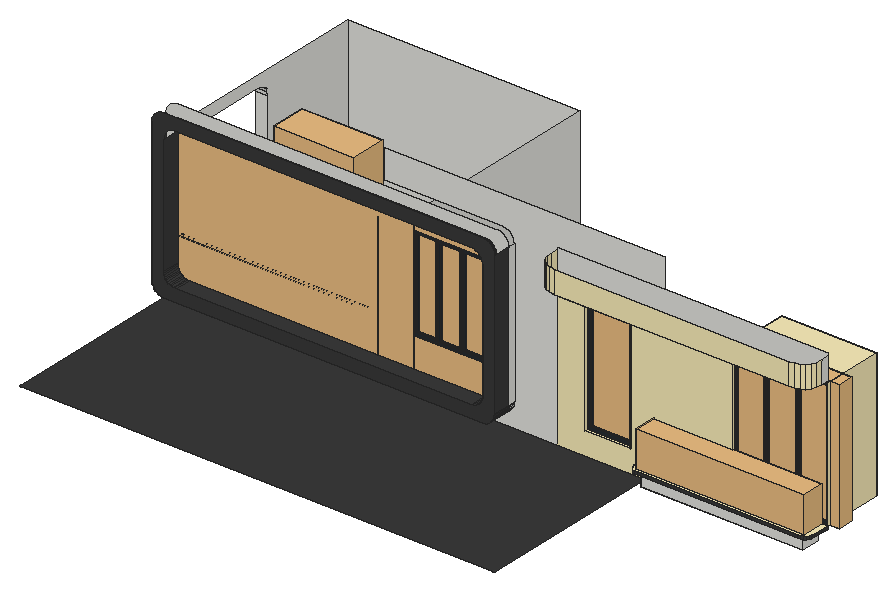
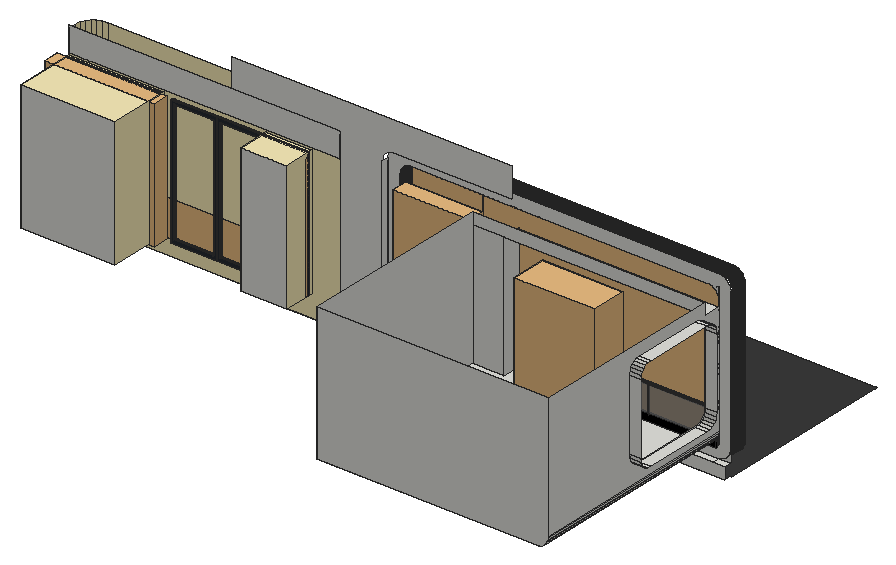
# SketchUp Ruby script. Lengths in inches.
U = 1.inch
M = Sketchup.active_model
def pt(a) = Geom::Point3d.new(a.map { |v| v * U })
def face(e, loops, mat)
  f = e.add_face(loops[0].map { |a| pt(a) })
  loops[1..].each { |l| e.add_face(l.map { |a| pt(a) }).erase! }
  f.material = f.back_material = mat if mat
  f
end
# faces: each face lists its corners as indices into pts; further lists are holes
def faces(e, pts, list, mat = nil) = list.each { |f| face(e, (f[0].is_a?(Array) ? f : [f]).map { |l| l.map { |i| pts[i] } }, mat) }
# xy, xz, yz: faces in a plane at the given z, y or x. An outline is a flat list of corners, or four numbers for a rectangle; further outlines are holes
def ring(l) = l.size == 4 ? [[l[0], l[1]], [l[2], l[1]], [l[2], l[3]], [l[0], l[3]]] : l.each_slice(2).to_a
def flat(e, list, mat, &to3) = list.each { |f| face(e, (f[0].is_a?(Array) ? f : [f]).map { |l| ring(l).map { |u, v| to3.(u, v) } }, mat) }
def xy(e, z, list, mat = nil) = flat(e, list, mat) { |x, y| [x, y, z] }
def xz(e, y, list, mat = nil) = flat(e, list, mat) { |x, z| [x, y, z] }
def yz(e, x, list, mat = nil) = flat(e, list, mat) { |y, z| [x, y, z] }
def lines(e, pts, list) = list.each { |a, b| e.add_line(pt(pts[a]), pt(pts[b])) }
# prism: a flat outline (further loops are holes) pulled along v
def prism(e, loops, v, mat = nil)
  f = face(e, loops, mat); d = Geom::Vector3d.new(v.map { |x| x * U })
  f.pushpull(f.normal.samedirection?(d) ? d.length : -d.length)
end
def box(e, o, s, mat = nil) = prism(e, [[o, [o[0] + s[0], o[1], o[2]], [o[0] + s[0], o[1] + s[1], o[2]], [o[0], o[1] + s[1], o[2]]]], [0, 0, s[2]], mat)
def at(x, y, z, deg = 0) = Geom::Transformation.translation(pt([x, y, z])) * Geom::Transformation.rotation(ORIGIN, Z_AXIS, deg.degrees)
def axes(o, x, y, z) = Geom::Transformation.new([*x, 0, *y, 0, *z, 0, *pt(o).to_a, 1])
def part(name) = M.definitions.add(name)
# library, detail: a bought-in or finely detailed component or shape, given as its bounding box
def library(name, o, s) = part(name).tap { |d| box(d.entities, o, s) }
def detail(e, o, s) = box(e.add_group.entities, o, s)
def put(e, d, t, mat = nil) = e.add_instance(d, t).tap { |i| i.material = mat if mat }
def group(e, t, mat = nil) = e.add_group.tap { |g| g.transformation = t; g.material = mat if mat }.entities
root = M.entities
M.materials.add("0899 AP 7833 SUNKISSED").color = [249, 236, 185]
M.materials.add("Glass Railing Color").color = [198, 198, 198]
M.materials.add("Railing Glass").color = [63, 150, 137]
M.materials["Railing Glass"].alpha = 0.13
M.materials.add("Wine2").color = [0, 0, 0]
M.materials["Wine2"].alpha = 0
M.materials.add("[0130_Gainsboro]").color = [39, 45, 50]
M.materials.add("[Color M07]").color = [58, 58, 58]
M.materials.add("[Color M09]").color = [0, 0, 0]
M.materials.add("[Translucent Glass Gray]").color = [128, 128, 128]
M.materials["[Translucent Glass Gray]"].alpha = 0.5
M.materials.add("[Wood Veneer 02]").color = [190, 128, 91]
c1 = part("Window sash")
xy(c1.entities,0,[[0,-0.98,43.07,0],[0,0,43.07,1.4]],"[0130_Gainsboro]")
xy(c1.entities,0.3,[[0.3,-1.43,42.77,-0.98]],"[0130_Gainsboro]")
xy(c1.entities,2.95,[[2.95,-1.43,40.12,-0.63],[2.95,-0.63,40.12,0],[2.95,0,40.12,0.64],[2.95,0.64,40.12,1.4]],"[0130_Gainsboro]")
xy(c1.entities,3.54,[[3.54,-0.63,39.53,0],[3.54,0,39.53,0.64]],"[0130_Gainsboro]")
xy(c1.entities,111.8125,[[3.54,-0.63,39.53,0],[3.54,0,39.53,0.64]],"[0130_Gainsboro]")
xy(c1.entities,112.4,[[2.95,-1.43,40.12,-0.63],[2.95,-0.63,40.12,0],[2.95,0,40.12,0.64],[2.95,0.64,40.12,1.4]],"[0130_Gainsboro]")
xy(c1.entities,115.05,[[0.3,-1.43,42.77,-0.98]],"[0130_Gainsboro]")
xy(c1.entities,115.35,[[0,-0.98,43.07,0],[0,0,43.07,1.4]],"[0130_Gainsboro]")
xz(c1.entities,-1.43,[[[0.3,0.3,42.77,115.05],[2.95,2.95,40.12,112.4]]],"[0130_Gainsboro]")
xz(c1.entities,-0.98,[[[0,0,43.07,115.35],[0.3,0.3,42.77,115.05]]],"[0130_Gainsboro]")
xz(c1.entities,-0.63,[[[2.95,2.95,40.12,112.4],[3.54,3.54,39.53,111.8125]]],"[0130_Gainsboro]")
xz(c1.entities,0,[[3.54,3.54,39.53,111.8125]],"Wine2")
xz(c1.entities,0,[[[0,0,43.07,115.35],[2.95,2.95,40.12,112.4]],[[2.95,2.95,40.12,112.4],[3.54,3.54,39.53,111.8125]]],"[0130_Gainsboro]")
xz(c1.entities,0.64,[[[2.95,2.95,40.12,112.4],[3.54,3.54,39.53,111.8125]]],"[0130_Gainsboro]")
xz(c1.entities,1.4,[[[0,0,43.07,115.35],[2.95,2.95,40.12,112.4]]],"[0130_Gainsboro]")
yz(c1.entities,0,[[-0.98,0,0,115.35],[0,0,1.4,115.35]],"[0130_Gainsboro]")
yz(c1.entities,0.3,[[-1.43,0.3,-0.98,115.05]],"[0130_Gainsboro]")
yz(c1.entities,2.95,[[-1.43,2.95,-0.63,112.4],[-0.63,2.95,0,112.4],[0,2.95,0.64,112.4],[0.64,2.95,1.4,112.4]],"[0130_Gainsboro]")
yz(c1.entities,3.54,[[-0.63,3.54,0,111.8125],[0,3.54,0.64,111.8125]],"[0130_Gainsboro]")
yz(c1.entities,39.53,[[-0.63,3.54,0,111.8125],[0,3.54,0.64,111.8125]],"[0130_Gainsboro]")
yz(c1.entities,40.12,[[-1.43,2.95,-0.63,112.4],[-0.63,2.95,0,112.4],[0,2.95,0.64,112.4],[0.64,2.95,1.4,112.4]],"[0130_Gainsboro]")
yz(c1.entities,42.77,[[-1.43,0.3,-0.98,115.05]],"[0130_Gainsboro]")
yz(c1.entities,43.07,[[-0.98,0,0,115.35],[0,0,1.4,115.35]],"[0130_Gainsboro]")
c2 = part("Three-panel window")
put(c2.entities,c1,axes([90.57,1.43,0],[1.05148,0,0],[0,1,0],[0,0,1]))
put(c2.entities,c1,axes([0,1.43,0],[1.05148,0,0],[0,1,0],[0,0,1]))
put(c2.entities,c1,axes([45.29,1.43,0],[1.05148,0,0],[0,1,0],[0,0,1]))
c3 = library("шторы раздвинутые\#1",[23.6875,-79.37,-3.6],[68.3125,79.85,10.87])
c4 = library("Glass Railing",[-110.8125,-14.6875,0],[111.5625,15.1875,24])
c5 = part("Group\#61")
p = [[0,1.89,0.38],[0,1.89,1.61],[0,0.72,0],[0,0,0.99],[0,0.72,1.99]]
lines(c5.entities,p,[[0,1],[2,0],[3,2],[4,3],[1,4]])
c6 = part("Pleated curtain panel")
p = [[20.45,2.26,80],[20.78,2.41,80]]
lines(c6.entities,p,[[0,1]])
detail(c6.entities,[0,1.93,2.7],[20.05,3.87,77.3])
put(c6.entities,c5,at(9.77,5.02,80,-180))
put(c6.entities,c5,at(11.91,5.02,80,-180))
put(c6.entities,c5,at(13.54,5.02,80,-180))
put(c6.entities,c5,at(7.29,5.02,80,-180))
put(c6.entities,c5,at(6.18,5.02,80,-180))
put(c6.entities,c5,at(8.69,5.02,80,-180))
put(c6.entities,c5,at(17.42,5.04,80,-180))
put(c6.entities,c5,at(18.86,5.04,80,-180))
put(c6.entities,c5,at(15.09,5.02,80,-180))
put(c6.entities,c5,at(16.66,5.04,80,-180))
put(c6.entities,c5,at(2.54,5.02,80,-180))
put(c6.entities,c5,at(1.38,5.02,80,-180))
put(c6.entities,c5,at(4.1,5.02,80,-180))
c7 = part("Glass Rail Spacer")
box(c7.entities,[-0.5,-0.25,0],[1,0.5,1],"Glass Railing Color")
c8 = part("Group19\#1")
prism(c8.entities,[[[0.54,0,1.27],[0.38,0,1.39],[0.21,0,1.47],[0.01,0,1.5],[-0.18,0,1.48],[-0.37,0,1.41],[-0.52,0,1.29],[-0.64,0,1.13],[-0.72,0,0.96],[-0.75,0,0.76],[-0.73,0,0.57],[-0.66,0,0.38],[-0.54,0,0.23],[-0.38,0,0.11],[-0.21,0,0.03],[-0.01,0,0],[0.18,0,0.02],[0.37,0,0.09],[0.52,0,0.21],[0.64,0,0.37],[0.72,0,0.54],[0.75,0,0.74],[0.73,0,0.93],[0.66,0,1.12]]],[0,136.79,0],"[Color M09]")
c9 = part("Group22\#2")
prism(c9.entities,[[[0.25,0,5],[0.25,0,4],[-0.25,0,4],[-0.25,0,5],[-0.5,0,5],[-0.5,0,0],[0.5,0,0],[0.5,0,5]]],[0,136.79,0],"[Color M09]")
c10 = part("Group23\#2")
box(c10.entities,[-0.1875,0,0],[0.375,44.26,18.5],"[Translucent Glass Gray]")
c11 = part("Group24\#2")
box(c11.entities,[-0.1875,0,0],[0.375,44.26,18.5],"[Translucent Glass Gray]")
c12 = part("Group25\#2")
box(c12.entities,[-0.1875,0,0],[0.375,44.26,18.5],"[Translucent Glass Gray]")
c13 = part("Glass Railing\#2")
put(c13.entities,c7,at(0,0,4,180))
put(c13.entities,c7,at(-45.26,0,4,180))
put(c13.entities,c7,at(-90.53,0,4,180))
put(c13.entities,c7,at(-135.79,0,4,180))
put(c13.entities,c8,at(0.5,0,22.5,90),"[Color M09]")
put(c13.entities,c9,at(0.5,0,0,90),"Glass Railing Color")
put(c13.entities,c10,at(-0.5,0,4,90),"[Translucent Glass Gray]")
put(c13.entities,c11,at(-45.76,0,4,90),"Railing Glass")
put(c13.entities,c12,at(-91.03,0,4,90),"Railing Glass")
c14 = library("Group24\#3",[-80,-48,0],[160,96,0.25])
c15 = library("Group160\#2",[-28,-10,0],[56,20,0.25])
c16 = library("sWING-1250",[0,0,16],[54.55,24,105.18])
c17 = part("Group253\#1")
prism(c17.entities,[[[-3,37.93,0],[-3,-38,0],[-4,-38,0],[-4,26,0],[-4,38,0]]],[0,0,0.25])
c18 = part("Group254\#1")
xy(c18.entities,0,[[-2.8125,-38,-2.8125,37.9,-1.93,37.73,-1.8125,37.6875,-1.8125,-38]])
xy(c18.entities,0.25,[[-2.8125,-38,-1.8125,-38,-1.8125,37.6875,-1.93,37.73,-2.8125,37.9]])
xz(c18.entities,-38,[[-2.8125,0,-1.8125,0.25]])
yz(c18.entities,-2.8125,[[-38,0,37.9,0.25]])
yz(c18.entities,-1.8125,[[-38,0,37.6875,0.25]])
c19 = part("Group255\#1")
xy(c19.entities,0,[[-1.625,-38,-1.625,37.625,-0.9375,37.39,-0.625,37.24,-0.625,-38]])
xy(c19.entities,0.25,[[-1.625,-38,-0.625,-38,-0.625,37.24,-0.9375,37.39,-1.625,37.625]])
xz(c19.entities,-38,[[-1.625,0,-0.625,0.25]])
yz(c19.entities,-1.625,[[-38,0,37.625,0.25]])
yz(c19.entities,-0.625,[[-38,0,37.24,0.25]])
c20 = part("Group256\#1")
xy(c20.entities,0,[[-0.4375,-38,-0.4375,37.14,0,36.93,0.5625,36.55,0.5625,-38]])
xy(c20.entities,0.25,[[-0.4375,-38,0.5625,-38,0.5625,36.55,0,36.93,-0.4375,37.14]])
xz(c20.entities,-38,[[-0.4375,0,0.5625,0.25]])
yz(c20.entities,-0.4375,[[-38,0,37.14,0.25]])
yz(c20.entities,0.5625,[[-38,0,36.55,0.25]])
c21 = part("Group257\#1")
xy(c21.entities,0,[[0.75,-38,0.75,36.43,0.87,36.35,1.66,35.66,1.75,35.55,1.75,-38]])
xy(c21.entities,0.25,[[0.75,-38,1.75,-38,1.75,35.55,1.66,35.66,0.87,36.35,0.75,36.43]])
xz(c21.entities,-38,[[0.75,0,1.75,0.25]])
yz(c21.entities,0.75,[[-38,0,36.43,0.25]])
yz(c21.entities,1.75,[[-38,0,35.55,0.25]])
c22 = part("Group258\#1")
xy(c22.entities,0,[[1.9375,-38,1.9375,35.34,2.35,34.87,2.93,34,2.9375,33.98,2.9375,-38]])
xy(c22.entities,0.25,[[1.9375,-38,2.9375,-38,2.9375,33.98,2.93,34,2.35,34.87,1.9375,35.34]])
yz(c22.entities,1.9375,[[-38,0,35.34,0.25]])
yz(c22.entities,2.9375,[[-38,0,33.98,0.25]])
c23 = part("Group259\#1")
xy(c23.entities,0,[[3.125,-38,3.125,33.6,3.39,33.0625,3.73,32.07,3.93,31.04,4,30,4,-38]])
xy(c23.entities,0.25,[[3.125,-38,4,-38,4,30,3.93,31.04,3.73,32.07,3.39,33.0625,3.125,33.6]])
yz(c23.entities,3.125,[[-38,0,33.6,0.25]])
c24 = part("Group251\#2")
put(c24.entities,c17,at(0,0,0))
put(c24.entities,c18,at(0,0,0))
put(c24.entities,c19,at(0,0,0))
put(c24.entities,c20,at(0,0,0))
put(c24.entities,c21,at(0,0,0))
put(c24.entities,c22,at(0,0,0))
put(c24.entities,c23,at(0,0,0))
c25 = library("Group209\#2",[-24,-6,0],[48,12,0.25])
xy(root,135,[[2.06,0,319.94,0,320.57,0.06,321.09,0.23,321.49,0.51,321.77,0.91,321.94,1.43,322,2.06,322,123.1875,321,123.1875,321,128.1875,1,128.1875,1,123.1875,0,123.1875,0,2.06,0.06,1.43,0.23,0.91,0.51,0.51,0.91,0.23,1.43,0.06],[321,123.1875,322,128.1875]],"[Color M07]")
xy(root,139,[[329.02,115.4375,438.6,128.1875]])
xy(root,143,[[1,123.1875,9,128.1875],[9,123.1875,225,128.1875]])
xy(root,143,[[9,111.1875,225,123.1875]],"[Color M07]")
xy(root,148,[[330.04,111.1875,328.1,111.36,326.51,111.89,325.28,112.78,324.39,114.01,323.92,115.4375,323.86,115.6,323.6875,117.54,323.6875,128.1875,329.02,128.1875,329.02,115.4375,444.77,115.4375,444.29,114.01,443.41,112.78,442.18,111.89,440.59,111.36,438.65,111.1875]])
xy(root,150,[[330.04,111.1875,438.65,111.1875,440.59,111.36,442.18,111.89,443.41,112.78,444.29,114.01,444.77,115.4375,444.82,115.6,445,117.54,445,128.1875,438.6,128.1875,438.6,115.4375,329.02,115.4375,329.02,128.1875,323.6875,128.1875,323.6875,117.54,323.86,115.6,323.92,115.4375,324.39,114.01,325.28,112.78,326.51,111.89,328.1,111.36],[280.5,128.1875,311.5,149.5],[380.875,128.1875,445,169.5625]],"0899 AP 7833 SUNKISSED")
xy(root,151,[[17,123.1875,144.79,123.1875,144.79,135.1875,166.1,135.1875,166.1,267.1875,17,267.1875]])
xy(root,151,[[17,111.1875,217,123.1875]],"[Color M07]")
xy(root,171,[[169,123.1875,217,132.9375],[1,143.3,9,191.01]])
xy(root,235,[[9,123.1875,144.79,135.1875],[169,123.1875,217,132.9375],[1,143.3,9,191.01]])
xy(root,236.98,[[280.5,128.1875,311.5,149.5],[380.875,128.1875,445,169.5625]],"0899 AP 7833 SUNKISSED")
xy(root,238,[[274.28,111.1875,270.45,111.52,267.32,112.52,264.88,114.1875,263.14,116.52,262.1,119.52,261.75,123.1875,261.75,128.1875,445,128.1875,445,123.1875,444.65,119.52,443.61,116.52,441.87,114.1875,439.43,112.52,436.3,111.52,432.47,111.1875]],"0899 AP 7833 SUNKISSED")
xz(root,111.1875,[[274.28,238,432.47,253.0625]],"0899 AP 7833 SUNKISSED")
xz(root,111.1875,[[[9,143,225,143,226.04,143.07,227.07,143.27,228.0625,143.61,229,144.07,229.87,144.65,230.66,145.34,231.35,146.13,231.93,147,232.39,147.9375,232.73,148.93,232.93,149.96,233,151,233,247,232.93,248.04,232.73,249.07,232.39,250.0625,231.93,251,231.35,251.87,230.66,252.66,229.87,253.35,229,253.93,228.0625,254.39,227.07,254.73,226.04,254.93,225,255,9,255,7.96,254.93,6.93,254.73,5.9375,254.39,5,253.93,4.13,253.35,3.34,252.66,2.65,251.87,2.07,251,1.61,250.0625,1.27,249.07,1.07,248.04,1,247,1,151,1.07,149.96,1.27,148.93,1.61,147.9375,2.07,147,2.65,146.13,3.34,145.34,4.13,144.65,5,144.07,5.9375,143.61,6.93,143.27,7.96,143.07],[17,151,15.96,151.07,14.93,151.27,13.9375,151.61,13,152.07,12.13,152.65,11.34,153.34,10.65,154.13,10.07,155,9.61,155.9375,9.27,156.93,9.07,157.96,9,159,9,239,9.07,240.04,9.27,241.07,9.61,242.0625,10.07,243,10.65,243.87,11.34,244.66,12.13,245.35,13,245.93,13.9375,246.39,14.93,246.73,15.96,246.93,17,247,217,247,218.04,246.93,219.07,246.73,220.0625,246.39,221,245.93,221.87,245.35,222.66,244.66,223.35,243.87,223.93,243,224.39,242.0625,224.73,241.07,224.93,240.04,225,239,225,159,224.93,157.96,224.73,156.93,224.39,155.9375,223.93,155,223.35,154.13,222.66,153.34,221.87,152.65,221,152.07,220.0625,151.61,219.07,151.27,218.04,151.07,217,151]],[330.04,148,438.65,150]],"[Color M07]")
xz(root,115.4375,[[329.02,139,438.6,148],[329.02,148,438.6,150]])
xz(root,123.1875,[[1,143,9,143,7.96,143.07,6.93,143.27,5.9375,143.61,5,144.07,4.13,144.65,3.34,145.34,2.65,146.13,2.07,147,1.61,147.9375,1.27,148.93,1.07,149.96,1,151],[[9,143,7.96,143.07,6.93,143.27,5.9375,143.61,5,144.07,4.13,144.65,3.34,145.34,2.65,146.13,2.07,147,1.61,147.9375,1.27,148.93,1.07,149.96,1,151,1,247,1.07,248.04,1.27,249.07,1.61,250.0625,2.07,251,2.65,251.87,3.34,252.66,4.13,253.35,5,253.93,5.9375,254.39,6.93,254.73,7.96,254.93,9,255,225,255,226.04,254.93,227.07,254.73,228.0625,254.39,229,253.93,229.87,253.35,230.66,252.66,231.35,251.87,231.93,251,232.39,250.0625,232.73,249.07,232.93,248.04,233,247,233,151,232.93,149.96,232.73,148.93,232.39,147.9375,231.93,147,231.35,146.13,230.66,145.34,229.87,144.65,229,144.07,228.0625,143.61,227.07,143.27,226.04,143.07,225,143],[17,151,217,151,218.04,151.07,219.07,151.27,220.0625,151.61,221,152.07,221.87,152.65,222.66,153.34,223.35,154.13,223.93,155,224.39,155.9375,224.73,156.93,224.93,157.96,225,159,225,239,224.93,240.04,224.73,241.07,224.39,242.0625,223.93,243,223.35,243.87,222.66,244.66,221.87,245.35,221,245.93,220.0625,246.39,219.07,246.73,218.04,246.93,217,247,17,247,15.96,246.93,14.93,246.73,13.9375,246.39,13,245.93,12.13,245.35,11.34,244.66,10.65,243.87,10.07,243,9.61,242.0625,9.27,241.07,9.07,240.04,9,239,9,159,9.07,157.96,9.27,156.93,9.61,155.9375,10.07,155,10.65,154.13,11.34,153.34,12.13,152.65,13,152.07,13.9375,151.61,14.93,151.27,15.96,151.07]]])
xz(root,128.1875,[[1,135,261.75,135,261.75,255,334.71,255,334.71,274.625,145.5625,274.625,145.5625,255,225,255,226.04,254.93,227.07,254.73,228.0625,254.39,229,253.93,229.87,253.35,230.66,252.66,231.35,251.87,231.93,251,232.39,250.0625,232.73,249.07,232.93,248.04,233,247,233,151,232.93,149.96,232.73,148.93,232.39,147.9375,231.93,147,231.35,146.13,230.66,145.34,229.87,144.65,229,144.07,228.0625,143.61,227.07,143.27,226.04,143.07,225,143,1,143],[323.6875,148,329.02,150],[261.75,238,445,255]])
xz(root,128.1875,[[[261.75,135,323.6875,135,323.6875,150,329.02,150,329.02,139,438.6,139,438.6,150,380.875,150,380.875,236.98,445,236.98,445,238,261.75,238],[280.5,150,311.5,236.98]]],"0899 AP 7833 SUNKISSED")
xz(root,132.9375,[[169,171,217,235]])
xz(root,135.1875,[[144.79,151,166.1,235],[1,179.11,9,226.89],[9,235,166.1,243]])
xz(root,149.5,[[280.5,150,311.5,236.98]])
xz(root,169.5625,[[380.875,150,445,236.98]])
xz(root,199.125,[[1,179.11,9,226.89]])
xz(root,267.1875,[[17,151,166.1,151,166.1,243,9,243,9,159,9.07,157.96,9.27,156.93,9.61,155.9375,10.07,155,10.65,154.13,11.34,153.34,12.13,152.65,13,152.07,13.9375,151.61,14.93,151.27,15.96,151.07]])
yz(root,1,[[111.1875,151,123.1875,247]],"[Color M07]")
yz(root,9,[[[123.1875,159,267.1875,159,267.1875,243,135.1875,243,135.1875,235,123.1875,235],[143.3,171,140.82,171.23,138.79,171.9,137.22,173.03,136.09,174.61,135.41,176.63,135.1875,179.11,135.1875,226.89,135.41,229.37,136.09,231.39,137.22,232.97,138.79,234.1,140.82,234.77,143.3,235,191.01,235,193.49,234.77,195.52,234.1,197.1,232.97,198.22,231.39,198.9,229.37,199.125,226.89,199.125,179.11,198.9,176.63,198.22,174.61,197.1,173.03,195.52,171.9,193.49,171.23,191.01,171]]])
yz(root,9,[[111.1875,159,123.1875,239]],"[Color M07]")
yz(root,144.79,[[123.1875,151,135.1875,235]])
yz(root,166.1,[[135.1875,151,267.1875,243]])
yz(root,169,[[123.1875,171,132.9375,235]])
yz(root,217,[[123.1875,171,132.9375,235]])
yz(root,225,[[111.1875,159,123.1875,239]],"[Color M07]")
yz(root,233,[[123.1875,151,128.1875,247]])
yz(root,233,[[111.1875,151,123.1875,247]],"[Color M07]")
yz(root,261.75,[[123.1875,238,128.1875,253.0625]],"0899 AP 7833 SUNKISSED")
yz(root,280.5,[[128.1875,150,149.5,236.98]],"0899 AP 7833 SUNKISSED")
yz(root,311.5,[[128.1875,150,149.5,236.98]],"0899 AP 7833 SUNKISSED")
yz(root,323.6875,[[117.54,148,128.1875,150]],"[Color M07]")
yz(root,329.02,[[115.4375,139,128.1875,148],[115.4375,148,128.1875,150]])
yz(root,380.875,[[128.1875,150,169.5625,236.98]],"0899 AP 7833 SUNKISSED")
yz(root,438.6,[[115.4375,139,128.1875,150]])
yz(root,445,[[123.1875,238,128.1875,253.0625]])
yz(root,445,[[128.1875,150,169.5625,236.98]],"0899 AP 7833 SUNKISSED")
yz(root,445,[[117.54,148,123.1875,150],[123.1875,148.01,128.1875,150]],"[Color M07]")
p = [[7.96,123.1875,143.07],[9,123.1875,143],[9,111.1875,143],[7.96,111.1875,143.07],[225,123.1875,143],[226.04,123.1875,143.07],
  [226.04,111.1875,143.07],[225,111.1875,143],[225,128.1875,143],[226.04,128.1875,143.07],[6.93,123.1875,143.27],[6.93,111.1875,143.27],
  [227.07,123.1875,143.27],[227.07,111.1875,143.27],[227.07,128.1875,143.27],[5.9375,123.1875,143.61],[5.9375,111.1875,143.61],[228.0625,123.1875,143.61],
  [228.0625,111.1875,143.61],[228.0625,128.1875,143.61],[5,123.1875,144.07],[5,111.1875,144.07],[229,123.1875,144.07],[229,111.1875,144.07],
  [229,128.1875,144.07],[4.13,123.1875,144.65],[4.13,111.1875,144.65],[229.87,123.1875,144.65],[229.87,111.1875,144.65],[229.87,128.1875,144.65],
  [3.34,123.1875,145.34],[3.34,111.1875,145.34],[230.66,123.1875,145.34],[230.66,111.1875,145.34],[230.66,128.1875,145.34],[2.65,123.1875,146.13],
  [2.65,111.1875,146.13],[231.35,123.1875,146.13],[231.35,111.1875,146.13],[231.35,128.1875,146.13],[2.07,123.1875,147],[2.07,111.1875,147],
  [231.93,123.1875,147],[231.93,111.1875,147],[231.93,128.1875,147],[1.61,123.1875,147.9375],[1.61,111.1875,147.9375],[232.39,123.1875,147.9375],
  [232.39,111.1875,147.9375],[232.39,128.1875,147.9375],[1.27,123.1875,148.93],[1.27,111.1875,148.93],[232.73,123.1875,148.93],[232.73,111.1875,148.93],
  [232.73,128.1875,148.93],[330.04,111.1875,150],[328.1,111.36,150],[328.1,111.36,148],[330.04,111.1875,148],[440.59,111.36,150],
  [438.65,111.1875,150],[438.65,111.1875,148],[440.59,111.36,148],[326.51,111.89,150],[326.51,111.89,148],[442.18,111.89,150],
  [442.18,111.89,148],[325.28,112.78,150],[325.28,112.78,148],[443.41,112.78,150],[443.41,112.78,148],[324.39,114.01,150],
  [324.39,114.01,148],[444.29,114.01,150],[444.29,114.01,148],[323.92,115.4375,150],[323.92,115.4375,148],[444.77,115.4375,150],
  [444.77,115.4375,148],[323.86,115.6,150],[323.86,115.6,148],[444.82,115.6,148],[444.82,115.6,150],[323.6875,117.54,150],
  [323.6875,117.54,148],[445,117.54,148],[445,117.54,150],[1.07,123.1875,149.96],[1.07,111.1875,149.96],[232.93,123.1875,149.96],
  [232.93,111.1875,149.96],[232.93,128.1875,149.96],[1,123.1875,151],[1,111.1875,151],[233,123.1875,151],[233,111.1875,151],
  [233,128.1875,151],[17,123.1875,151],[15.96,123.1875,151.07],[15.96,111.1875,151.07],[17,111.1875,151],[218.04,123.1875,151.07],
  [217,123.1875,151],[217,111.1875,151],[218.04,111.1875,151.07],[17,267.1875,151],[15.96,267.1875,151.07],[14.93,123.1875,151.27],
  [14.93,111.1875,151.27],[219.07,123.1875,151.27],[219.07,111.1875,151.27],[14.93,267.1875,151.27],[13.9375,123.1875,151.61],[13.9375,111.1875,151.61],
  [220.0625,123.1875,151.61],[220.0625,111.1875,151.61],[13.9375,267.1875,151.61],[13,123.1875,152.07],[13,111.1875,152.07],[221,123.1875,152.07],
  [221,111.1875,152.07],[13,267.1875,152.07],[12.13,123.1875,152.65],[12.13,111.1875,152.65],[221.87,123.1875,152.65],[221.87,111.1875,152.65],
  [12.13,267.1875,152.65],[11.34,123.1875,153.34],[11.34,111.1875,153.34],[222.66,123.1875,153.34],[222.66,111.1875,153.34],[11.34,267.1875,153.34],
  [10.65,123.1875,154.13],[10.65,111.1875,154.13],[223.35,123.1875,154.13],[223.35,111.1875,154.13],[10.65,267.1875,154.13],[10.07,123.1875,155],
  [10.07,111.1875,155],[223.93,123.1875,155],[223.93,111.1875,155],[10.07,267.1875,155],[9.61,123.1875,155.9375],[9.61,111.1875,155.9375],
  [224.39,123.1875,155.9375],[224.39,111.1875,155.9375],[9.61,267.1875,155.9375],[9.27,123.1875,156.93],[9.27,111.1875,156.93],[224.73,123.1875,156.93],
  [224.73,111.1875,156.93],[9.27,267.1875,156.93],[9.07,123.1875,157.96],[9.07,111.1875,157.96],[224.93,123.1875,157.96],[224.93,111.1875,157.96],
  [9.07,267.1875,157.96],[9,123.1875,159],[9,111.1875,159],[225,123.1875,159],[225,111.1875,159],[9,267.1875,159],
  [1,140.82,171.23],[9,140.82,171.23],[9,143.3,171],[1,143.3,171],[1,191.01,171],[9,191.01,171],
  [9,193.49,171.23],[1,193.49,171.23],[1,138.79,171.9],[9,138.79,171.9],[9,195.52,171.9],[1,195.52,171.9],
  [1,137.22,173.03],[9,137.22,173.03],[9,197.1,173.03],[1,197.1,173.03],[1,136.09,174.61],[9,136.09,174.61],
  [9,198.22,174.61],[1,198.22,174.61],[1,135.41,176.63],[9,135.41,176.63],[9,198.9,176.63],[1,198.9,176.63],
  [1,135.1875,179.11],[9,135.1875,179.11],[9,199.125,179.11],[1,199.125,179.11],[1,135.41,229.37],[9,135.41,229.37],
  [9,135.1875,226.89],[1,135.1875,226.89],[1,199.125,226.89],[9,199.125,226.89],[9,198.9,229.37],[1,198.9,229.37],
  [1,136.09,231.39],[9,136.09,231.39],[9,198.22,231.39],[1,198.22,231.39],[1,137.22,232.97],[9,137.22,232.97],
  [9,197.1,232.97],[1,197.1,232.97],[1,138.79,234.1],[9,138.79,234.1],[9,195.52,234.1],[1,195.52,234.1],
  [1,140.82,234.77],[9,140.82,234.77],[9,193.49,234.77],[1,193.49,234.77],[1,143.3,235],[9,143.3,235],
  [9,191.01,235],[1,191.01,235],[270.45,111.52,238],[274.28,111.1875,238],[274.28,111.1875,253.0625],[270.45,111.52,253.0625],
  [432.47,111.1875,238],[436.3,111.52,238],[436.3,111.52,253.0625],[432.47,111.1875,253.0625],[267.32,112.52,238],[267.32,112.52,253.0625],
  [439.43,112.52,238],[439.43,112.52,253.0625],[264.88,114.1875,238],[264.88,114.1875,253.0625],[441.87,114.1875,238],[441.87,114.1875,253.0625],
  [263.14,116.52,238],[263.14,116.52,253.0625],[443.61,116.52,238],[443.61,116.52,253.0625],[262.1,119.52,238],[262.1,119.52,253.0625],
  [444.65,119.52,238],[444.65,119.52,253.0625],[261.75,123.1875,238],[261.75,123.1875,253.0625],[445,123.1875,238],[445,123.1875,253.0625],
  [169,123.1875,235],[169,123.1875,247],[169,123.1875,171],[169,123.1875,151],[217,123.1875,171],[225,123.1875,171],
  [217,123.1875,235],[217,123.1875,247]]
faces(root,p,[[0,1,2,3],[4,5,6,7],[10,0,3,11],[5,12,13,6],[15,10,11,16],[12,17,18,13],[20,15,16,21],[17,22,23,18],
  [25,20,21,26],[22,27,28,23],[30,25,26,31],[27,32,33,28],[35,30,31,36],[32,37,38,33],[40,35,36,41],[37,42,43,38],
  [45,40,41,46],[42,47,48,43],[50,45,46,51],[47,52,53,48],[55,56,57,58],[59,60,61,62],[56,63,64,57],[65,59,62,66],
  [63,67,68,64],[69,65,66,70],[67,71,72,68],[73,69,70,74],[71,75,76,72],[77,73,74,78],[75,79,80,76],[77,78,81,82],
  [79,83,84,80],[82,81,85,86],[87,50,51,88],[52,89,90,53],[92,87,88,93],[89,94,95,90],[97,98,99,100],[101,102,103,104],
  [98,107,108,99],[109,101,104,110],[107,112,113,108],[114,109,110,115],[112,117,118,113],[119,114,115,120],[117,122,123,118],[124,119,120,125],
  [122,127,128,123],[129,124,125,130],[127,132,133,128],[134,129,130,135],[132,137,138,133],[139,134,135,140],[137,142,143,138],[144,139,140,145],
  [142,147,148,143],[149,144,145,150],[147,152,153,148],[154,149,150,155],[152,157,158,153],[159,154,155,160]],"[Color M07]")
faces(root,p,[[5,4,8,9],[12,5,9,14],[17,12,14,19],[22,17,19,24],[27,22,24,29],[32,27,29,34],[37,32,34,39],[42,37,39,44],
  [47,42,44,49],[52,47,49,54],[89,52,54,91],[94,89,91,96],[98,97,105,106],[107,98,106,111],[112,107,111,116],[117,112,116,121],
  [122,117,121,126],[127,122,126,131],[132,127,131,136],[137,132,136,141],[142,137,141,146],[147,142,146,151],[152,147,151,156],[157,152,156,161],
  [162,163,164,165],[166,167,168,169],[170,171,163,162],[169,168,172,173],[174,175,171,170],[173,172,176,177],[178,179,175,174],[177,176,180,181],
  [182,183,179,178],[181,180,184,185],[186,187,183,182],[185,184,188,189],[190,191,192,193],[194,195,196,197],[198,199,191,190],[197,196,200,201],
  [202,203,199,198],[201,200,204,205],[206,207,203,202],[205,204,208,209],[210,211,207,206],[209,208,212,213],[214,215,211,210],[213,212,216,217]])
faces(root,p,[[218,219,220,221],[222,223,224,225],[226,218,221,227],[223,228,229,224],[230,226,227,231],[228,232,233,229],[234,230,231,235],[232,236,237,233],
  [238,234,235,239],[236,240,241,237],[242,238,239,243],[240,244,245,241]],"0899 AP 7833 SUNKISSED")
lines(root,p,[[246,247],[248,249],[250,251],[252,253]])
put(root,c2,axes([380.875,129.89,150],[0.47199,0,0],[0,0.4,0],[0,0,0.75403]))
put(root,c2,axes([280.5,130.54,150],[0.67965,0,0],[0,0.536,0],[0,0,0.75403]))
put(root,c3,axes([351.24,137.4375,236.46],[1.09,0,0],[0,0,1.08938],[0,-1,0]))
put(root,c4,axes([440.27,128.1875,150],[1.02,0,0],[0,1,0],[0,0,1]))
put(root,c6,axes([280.5,131.18,147.04],[1.49236,0,0],[0,0.36,0],[0,0,1.09705]))
put(root,c13,at(144.79,126.1,151))
put(root,c14,axes([89,123.1875,199],[1,0,0],[0,0,1],[0,-1,0]),"[Wood Veneer 02]")
put(root,c15,axes([197,123.1875,161],[1,0,0],[0,0,1],[0,-1,0]),"[Wood Veneer 02]")
put(root,c16,axes([49.87,153.37,156.55],[1,0,0],[0,1,0],[0,0,0.7134]))
put(root,c2,axes([169,123.1875,171],[0.3533,0,0],[0,1,0],[0,0,0.55499]))
put(root,c24,axes([221,123.1875,209],[1,0,0],[0,0,1],[0,-1,0]),"[Wood Veneer 02]")
put(root,c3,axes([149.02,132.66,237.67],[0.76595,0,0],[0,0,0.84006],[0,-1,0]))
put(root,c25,axes([193,123.1875,241],[1,0,0],[0,0,1],[0,-1,0]),"[Wood Veneer 02]")
